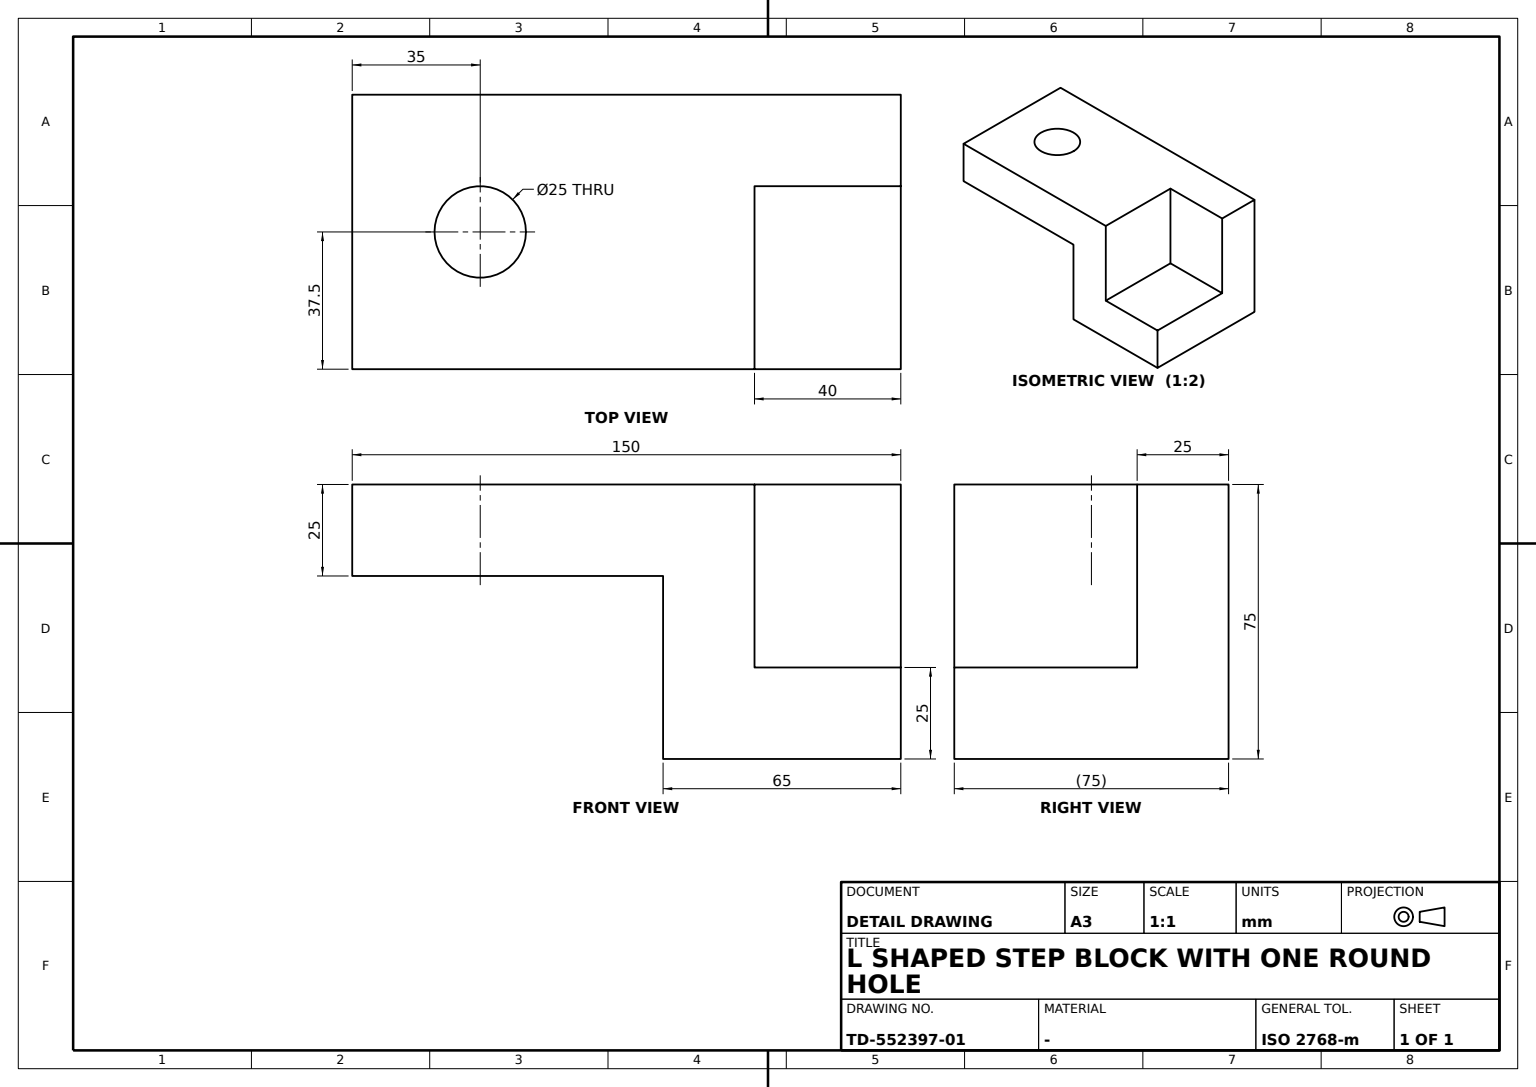
ISO-10303-21;
HEADER;
FILE_DESCRIPTION((''),'2;1');
FILE_NAME('','',(''),(''),'','','');
FILE_SCHEMA(('AUTOMOTIVE_DESIGN'));
ENDSEC;
DATA;
#10=SHAPE_REPRESENTATION_RELATIONSHIP('','',#262,#11);
#11=ADVANCED_BREP_SHAPE_REPRESENTATION('',(#260),#416);
#12=CIRCLE('',#268,12.5);
#13=CIRCLE('',#269,12.5);
#14=CIRCLE('',#274,12.5);
#15=CIRCLE('',#278,12.5);
#16=CYLINDRICAL_SURFACE('',#267,12.5);
#17=CYLINDRICAL_SURFACE('',#280,12.5);
#18=ORIENTED_EDGE('',*,*,#84,.F.);
#19=ORIENTED_EDGE('',*,*,#85,.F.);
#20=ORIENTED_EDGE('',*,*,#86,.T.);
#21=ORIENTED_EDGE('',*,*,#87,.T.);
#22=ORIENTED_EDGE('',*,*,#88,.T.);
#23=ORIENTED_EDGE('',*,*,#85,.T.);
#24=ORIENTED_EDGE('',*,*,#89,.T.);
#25=ORIENTED_EDGE('',*,*,#90,.F.);
#26=ORIENTED_EDGE('',*,*,#89,.F.);
#27=ORIENTED_EDGE('',*,*,#84,.T.);
#28=ORIENTED_EDGE('',*,*,#91,.F.);
#29=ORIENTED_EDGE('',*,*,#92,.F.);
#30=ORIENTED_EDGE('',*,*,#93,.F.);
#31=ORIENTED_EDGE('',*,*,#94,.F.);
#32=ORIENTED_EDGE('',*,*,#95,.F.);
#33=ORIENTED_EDGE('',*,*,#96,.F.);
#34=ORIENTED_EDGE('',*,*,#97,.F.);
#35=ORIENTED_EDGE('',*,*,#98,.F.);
#36=ORIENTED_EDGE('',*,*,#99,.F.);
#37=ORIENTED_EDGE('',*,*,#100,.F.);
#38=ORIENTED_EDGE('',*,*,#101,.F.);
#39=ORIENTED_EDGE('',*,*,#102,.F.);
#40=ORIENTED_EDGE('',*,*,#100,.T.);
#41=ORIENTED_EDGE('',*,*,#103,.F.);
#42=ORIENTED_EDGE('',*,*,#104,.F.);
#43=ORIENTED_EDGE('',*,*,#105,.T.);
#44=ORIENTED_EDGE('',*,*,#101,.T.);
#45=ORIENTED_EDGE('',*,*,#105,.F.);
#46=ORIENTED_EDGE('',*,*,#106,.F.);
#47=ORIENTED_EDGE('',*,*,#107,.T.);
#48=ORIENTED_EDGE('',*,*,#102,.T.);
#49=ORIENTED_EDGE('',*,*,#107,.F.);
#50=ORIENTED_EDGE('',*,*,#108,.F.);
#51=ORIENTED_EDGE('',*,*,#109,.T.);
#52=ORIENTED_EDGE('',*,*,#110,.T.);
#53=ORIENTED_EDGE('',*,*,#96,.T.);
#54=ORIENTED_EDGE('',*,*,#97,.T.);
#55=ORIENTED_EDGE('',*,*,#109,.F.);
#56=ORIENTED_EDGE('',*,*,#111,.F.);
#57=ORIENTED_EDGE('',*,*,#112,.T.);
#58=ORIENTED_EDGE('',*,*,#90,.T.);
#59=ORIENTED_EDGE('',*,*,#92,.T.);
#60=ORIENTED_EDGE('',*,*,#113,.T.);
#61=ORIENTED_EDGE('',*,*,#111,.T.);
#62=ORIENTED_EDGE('',*,*,#108,.T.);
#63=ORIENTED_EDGE('',*,*,#106,.T.);
#64=ORIENTED_EDGE('',*,*,#104,.T.);
#65=ORIENTED_EDGE('',*,*,#114,.T.);
#66=ORIENTED_EDGE('',*,*,#87,.F.);
#67=ORIENTED_EDGE('',*,*,#115,.T.);
#68=ORIENTED_EDGE('',*,*,#98,.T.);
#69=ORIENTED_EDGE('',*,*,#112,.F.);
#70=ORIENTED_EDGE('',*,*,#113,.F.);
#71=ORIENTED_EDGE('',*,*,#91,.T.);
#72=ORIENTED_EDGE('',*,*,#94,.T.);
#73=ORIENTED_EDGE('',*,*,#116,.T.);
#74=ORIENTED_EDGE('',*,*,#86,.F.);
#75=ORIENTED_EDGE('',*,*,#88,.F.);
#76=ORIENTED_EDGE('',*,*,#114,.F.);
#77=ORIENTED_EDGE('',*,*,#103,.T.);
#78=ORIENTED_EDGE('',*,*,#99,.T.);
#79=ORIENTED_EDGE('',*,*,#115,.F.);
#80=ORIENTED_EDGE('',*,*,#116,.F.);
#81=ORIENTED_EDGE('',*,*,#93,.T.);
#82=ORIENTED_EDGE('',*,*,#110,.F.);
#83=ORIENTED_EDGE('',*,*,#95,.T.);
#84=EDGE_CURVE('',#117,#118,#139,.T.);
#85=EDGE_CURVE('',#119,#117,#140,.T.);
#86=EDGE_CURVE('',#119,#120,#141,.T.);
#87=EDGE_CURVE('',#120,#118,#142,.T.);
#88=EDGE_CURVE('',#121,#119,#143,.T.);
#89=EDGE_CURVE('',#117,#122,#144,.T.);
#90=EDGE_CURVE('',#121,#122,#145,.T.);
#91=EDGE_CURVE('',#123,#118,#146,.T.);
#92=EDGE_CURVE('',#122,#123,#147,.T.);
#93=EDGE_CURVE('',#124,#125,#148,.T.);
#94=EDGE_CURVE('',#126,#124,#12,.T.);
#95=EDGE_CURVE('',#127,#126,#149,.F.);
#96=EDGE_CURVE('',#125,#127,#13,.T.);
#97=EDGE_CURVE('',#128,#129,#150,.T.);
#98=EDGE_CURVE('',#130,#128,#151,.T.);
#99=EDGE_CURVE('',#131,#130,#152,.T.);
#100=EDGE_CURVE('',#132,#131,#153,.T.);
#101=EDGE_CURVE('',#133,#132,#154,.T.);
#102=EDGE_CURVE('',#129,#133,#155,.T.);
#103=EDGE_CURVE('',#134,#131,#156,.T.);
#104=EDGE_CURVE('',#135,#134,#157,.T.);
#105=EDGE_CURVE('',#135,#132,#158,.T.);
#106=EDGE_CURVE('',#136,#135,#159,.T.);
#107=EDGE_CURVE('',#136,#133,#160,.T.);
#108=EDGE_CURVE('',#137,#136,#161,.T.);
#109=EDGE_CURVE('',#137,#129,#162,.T.);
#110=EDGE_CURVE('',#127,#125,#14,.T.);
#111=EDGE_CURVE('',#138,#137,#163,.T.);
#112=EDGE_CURVE('',#138,#128,#164,.T.);
#113=EDGE_CURVE('',#123,#138,#165,.T.);
#114=EDGE_CURVE('',#134,#121,#166,.T.);
#115=EDGE_CURVE('',#120,#130,#167,.T.);
#116=EDGE_CURVE('',#124,#126,#15,.T.);
#117=VERTEX_POINT('',#349);
#118=VERTEX_POINT('',#350);
#119=VERTEX_POINT('',#352);
#120=VERTEX_POINT('',#354);
#121=VERTEX_POINT('',#358);
#122=VERTEX_POINT('',#360);
#123=VERTEX_POINT('',#364);
#124=VERTEX_POINT('',#368);
#125=VERTEX_POINT('',#369);
#126=VERTEX_POINT('',#371);
#127=VERTEX_POINT('',#373);
#128=VERTEX_POINT('',#377);
#129=VERTEX_POINT('',#378);
#130=VERTEX_POINT('',#380);
#131=VERTEX_POINT('',#382);
#132=VERTEX_POINT('',#384);
#133=VERTEX_POINT('',#386);
#134=VERTEX_POINT('',#390);
#135=VERTEX_POINT('',#392);
#136=VERTEX_POINT('',#396);
#137=VERTEX_POINT('',#400);
#138=VERTEX_POINT('',#405);
#139=LINE('',#348,#168);
#140=LINE('',#351,#169);
#141=LINE('',#353,#170);
#142=LINE('',#355,#171);
#143=LINE('',#357,#172);
#144=LINE('',#359,#173);
#145=LINE('',#361,#174);
#146=LINE('',#363,#175);
#147=LINE('',#365,#176);
#148=LINE('',#367,#177);
#149=LINE('',#372,#178);
#150=LINE('',#376,#179);
#151=LINE('',#379,#180);
#152=LINE('',#381,#181);
#153=LINE('',#383,#182);
#154=LINE('',#385,#183);
#155=LINE('',#387,#184);
#156=LINE('',#389,#185);
#157=LINE('',#391,#186);
#158=LINE('',#393,#187);
#159=LINE('',#395,#188);
#160=LINE('',#397,#189);
#161=LINE('',#399,#190);
#162=LINE('',#401,#191);
#163=LINE('',#404,#192);
#164=LINE('',#406,#193);
#165=LINE('',#408,#194);
#166=LINE('',#409,#195);
#167=LINE('',#411,#196);
#168=VECTOR('',#285,1000.);
#169=VECTOR('',#286,1000.);
#170=VECTOR('',#287,1000.);
#171=VECTOR('',#288,1000.);
#172=VECTOR('',#291,1000.);
#173=VECTOR('',#292,1000.);
#174=VECTOR('',#293,1000.);
#175=VECTOR('',#296,1000.);
#176=VECTOR('',#297,1000.);
#177=VECTOR('',#300,1000.);
#178=VECTOR('',#303,1000.);
#179=VECTOR('',#308,1000.);
#180=VECTOR('',#309,1000.);
#181=VECTOR('',#310,1000.);
#182=VECTOR('',#311,1000.);
#183=VECTOR('',#312,1000.);
#184=VECTOR('',#313,1000.);
#185=VECTOR('',#316,1000.);
#186=VECTOR('',#317,1000.);
#187=VECTOR('',#318,1000.);
#188=VECTOR('',#321,1000.);
#189=VECTOR('',#322,1000.);
#190=VECTOR('',#325,1000.);
#191=VECTOR('',#326,1000.);
#192=VECTOR('',#331,1000.);
#193=VECTOR('',#332,1000.);
#194=VECTOR('',#335,1000.);
#195=VECTOR('',#336,1000.);
#196=VECTOR('',#339,1000.);
#197=EDGE_LOOP('',(#18,#19,#20,#21));
#198=EDGE_LOOP('',(#22,#23,#24,#25));
#199=EDGE_LOOP('',(#26,#27,#28,#29));
#200=EDGE_LOOP('',(#30,#31,#32,#33));
#201=EDGE_LOOP('',(#34,#35,#36,#37,#38,#39));
#202=EDGE_LOOP('',(#40,#41,#42,#43));
#203=EDGE_LOOP('',(#44,#45,#46,#47));
#204=EDGE_LOOP('',(#48,#49,#50,#51));
#205=EDGE_LOOP('',(#52,#53));
#206=EDGE_LOOP('',(#54,#55,#56,#57));
#207=EDGE_LOOP('',(#58,#59,#60,#61,#62,#63,#64,#65));
#208=EDGE_LOOP('',(#66,#67,#68,#69,#70,#71));
#209=EDGE_LOOP('',(#72,#73));
#210=EDGE_LOOP('',(#74,#75,#76,#77,#78,#79));
#211=EDGE_LOOP('',(#80,#81,#82,#83));
#212=FACE_BOUND('',#197,.T.);
#213=FACE_BOUND('',#198,.T.);
#214=FACE_BOUND('',#199,.T.);
#215=FACE_BOUND('',#200,.T.);
#216=FACE_BOUND('',#201,.T.);
#217=FACE_BOUND('',#202,.T.);
#218=FACE_BOUND('',#203,.T.);
#219=FACE_BOUND('',#204,.T.);
#220=FACE_BOUND('',#205,.T.);
#221=FACE_BOUND('',#206,.T.);
#222=FACE_BOUND('',#207,.T.);
#223=FACE_BOUND('',#208,.T.);
#224=FACE_BOUND('',#209,.T.);
#225=FACE_BOUND('',#210,.T.);
#226=FACE_BOUND('',#211,.T.);
#227=PLANE('',#264);
#228=PLANE('',#265);
#229=PLANE('',#266);
#230=PLANE('',#270);
#231=PLANE('',#271);
#232=PLANE('',#272);
#233=PLANE('',#273);
#234=PLANE('',#275);
#235=PLANE('',#276);
#236=PLANE('',#277);
#237=PLANE('',#279);
#238=ADVANCED_FACE('',(#212),#227,.T.);
#239=ADVANCED_FACE('',(#213),#228,.T.);
#240=ADVANCED_FACE('',(#214),#229,.T.);
#241=ADVANCED_FACE('',(#215),#16,.F.);
#242=ADVANCED_FACE('',(#216),#230,.F.);
#243=ADVANCED_FACE('',(#217),#231,.F.);
#244=ADVANCED_FACE('',(#218),#232,.F.);
#245=ADVANCED_FACE('',(#219,#220),#233,.F.);
#246=ADVANCED_FACE('',(#221),#234,.F.);
#247=ADVANCED_FACE('',(#222),#235,.T.);
#248=ADVANCED_FACE('',(#223,#224),#236,.F.);
#249=ADVANCED_FACE('',(#225),#237,.F.);
#250=ADVANCED_FACE('',(#226),#17,.F.);
#251=CLOSED_SHELL('',(#238,#239,#240,#241,#242,#243,#244,#245,#246,#247,#248,#249,#250));
#260=MANIFOLD_SOLID_BREP('',#251);
#261=SHAPE_DEFINITION_REPRESENTATION(#421,#262);
#262=SHAPE_REPRESENTATION('',(#263),#416);
#263=AXIS2_PLACEMENT_3D('',#346,#281,#282);
#264=AXIS2_PLACEMENT_3D('',#347,#283,#284);
#265=AXIS2_PLACEMENT_3D('',#356,#289,#290);
#266=AXIS2_PLACEMENT_3D('',#362,#294,#295);
#267=AXIS2_PLACEMENT_3D('',#366,#298,#299);
#268=AXIS2_PLACEMENT_3D('',#370,#301,#302);
#269=AXIS2_PLACEMENT_3D('',#374,#304,#305);
#270=AXIS2_PLACEMENT_3D('',#375,#306,#307);
#271=AXIS2_PLACEMENT_3D('',#388,#314,#315);
#272=AXIS2_PLACEMENT_3D('',#394,#319,#320);
#273=AXIS2_PLACEMENT_3D('',#398,#323,#324);
#274=AXIS2_PLACEMENT_3D('',#402,#327,#328);
#275=AXIS2_PLACEMENT_3D('',#403,#329,#330);
#276=AXIS2_PLACEMENT_3D('',#407,#333,#334);
#277=AXIS2_PLACEMENT_3D('',#410,#337,#338);
#278=AXIS2_PLACEMENT_3D('',#412,#340,#341);
#279=AXIS2_PLACEMENT_3D('',#413,#342,#343);
#280=AXIS2_PLACEMENT_3D('',#414,#344,#345);
#281=DIRECTION('',(0.,0.,1.));
#282=DIRECTION('',(1.,0.,0.));
#283=DIRECTION('',(0.,-1.,0.));
#284=DIRECTION('',(0.,0.,-1.));
#285=DIRECTION('',(0.,0.,1.));
#286=DIRECTION('',(-1.,0.,0.));
#287=DIRECTION('',(0.,0.,1.));
#288=DIRECTION('',(-1.,0.,0.));
#289=DIRECTION('',(0.,0.,1.));
#290=DIRECTION('',(1.,0.,0.));
#291=DIRECTION('',(0.,1.,0.));
#292=DIRECTION('',(0.,-1.,0.));
#293=DIRECTION('',(-1.,0.,0.));
#294=DIRECTION('',(1.,0.,0.));
#295=DIRECTION('',(0.,0.,-1.));
#296=DIRECTION('',(0.,1.,0.));
#297=DIRECTION('',(0.,0.,1.));
#298=DIRECTION('',(-9.25185853854297E-17,0.,-1.));
#299=DIRECTION('',(-1.,0.,0.));
#300=DIRECTION('',(-9.25185853854297E-17,0.,-1.));
#301=DIRECTION('',(-9.25185853854297E-17,0.,-1.));
#302=DIRECTION('',(-1.,0.,0.));
#303=DIRECTION('',(-9.25185853854297E-17,0.,-1.));
#304=DIRECTION('',(0.,0.,1.));
#305=DIRECTION('',(1.,0.,0.));
#306=DIRECTION('',(0.,-1.,0.));
#307=DIRECTION('',(0.,0.,-1.));
#308=DIRECTION('',(-1.11022302462516E-15,0.,-1.));
#309=DIRECTION('',(-1.,0.,9.25185853854297E-17));
#310=DIRECTION('',(-2.77555756156289E-17,0.,1.));
#311=DIRECTION('',(1.,0.,8.32667268468867E-17));
#312=DIRECTION('',(0.,0.,-1.));
#313=DIRECTION('',(1.,0.,0.));
#314=DIRECTION('',(-8.32667268468867E-17,0.,1.));
#315=DIRECTION('',(1.,0.,8.32667268468867E-17));
#316=DIRECTION('',(0.,1.,0.));
#317=DIRECTION('',(1.,0.,8.32667268468867E-17));
#318=DIRECTION('',(0.,1.,0.));
#319=DIRECTION('',(1.,0.,0.));
#320=DIRECTION('',(0.,0.,-1.));
#321=DIRECTION('',(0.,0.,-1.));
#322=DIRECTION('',(0.,1.,0.));
#323=DIRECTION('',(0.,0.,1.));
#324=DIRECTION('',(1.,0.,0.));
#325=DIRECTION('',(1.,0.,0.));
#326=DIRECTION('',(0.,1.,0.));
#327=DIRECTION('',(0.,0.,1.));
#328=DIRECTION('',(1.,0.,0.));
#329=DIRECTION('',(1.,0.,-1.11022302462516E-15));
#330=DIRECTION('',(-1.11022302462516E-15,0.,-1.));
#331=DIRECTION('',(-1.11022302462516E-15,0.,-1.));
#332=DIRECTION('',(0.,1.,0.));
#333=DIRECTION('',(0.,-1.,0.));
#334=DIRECTION('',(0.,0.,-1.));
#335=DIRECTION('',(-1.,0.,9.25185853854297E-17));
#336=DIRECTION('',(-2.77555756156289E-17,0.,1.));
#337=DIRECTION('',(-9.25185853854297E-17,0.,-1.));
#338=DIRECTION('',(-1.,0.,9.25185853854297E-17));
#339=DIRECTION('',(0.,1.,0.));
#340=DIRECTION('',(-9.25185853854297E-17,0.,-1.));
#341=DIRECTION('',(-1.,0.,0.));
#342=DIRECTION('',(-1.,0.,-2.77555756156289E-17));
#343=DIRECTION('',(-2.77555756156289E-17,0.,1.));
#344=DIRECTION('',(-9.25185853854297E-17,0.,-1.));
#345=DIRECTION('',(-1.,0.,0.));
#346=CARTESIAN_POINT('',(0.,0.,0.));
#347=CARTESIAN_POINT('',(0.,-25.,0.));
#348=CARTESIAN_POINT('',(-40.,-25.,75.));
#349=CARTESIAN_POINT('',(-40.,-25.,25.));
#350=CARTESIAN_POINT('',(-40.,-25.,75.));
#351=CARTESIAN_POINT('',(-40.,-25.,25.));
#352=CARTESIAN_POINT('',(0.,-25.,25.));
#353=CARTESIAN_POINT('',(-2.08166817117217E-15,-25.,25.));
#354=CARTESIAN_POINT('',(-2.08166817117217E-15,-25.,75.));
#355=CARTESIAN_POINT('',(0.,-25.,75.));
#356=CARTESIAN_POINT('',(-40.,-150.,25.));
#357=CARTESIAN_POINT('',(0.,-150.,25.));
#358=CARTESIAN_POINT('',(0.,-75.,25.));
#359=CARTESIAN_POINT('',(-40.,-150.,25.));
#360=CARTESIAN_POINT('',(-40.,-75.,25.));
#361=CARTESIAN_POINT('',(0.,-75.,25.));
#362=CARTESIAN_POINT('',(-40.,-150.,75.));
#363=CARTESIAN_POINT('',(-40.,-150.,75.));
#364=CARTESIAN_POINT('',(-40.,-75.,75.));
#365=CARTESIAN_POINT('',(-40.,-75.,0.));
#366=CARTESIAN_POINT('',(-115.,-37.5,75.));
#367=CARTESIAN_POINT('',(-102.5,-37.5,75.));
#368=CARTESIAN_POINT('',(-102.5,-37.5,75.));
#369=CARTESIAN_POINT('',(-102.5,-37.5,50.));
#370=CARTESIAN_POINT('',(-115.,-37.5,75.));
#371=CARTESIAN_POINT('',(-127.5,-37.5,75.));
#372=CARTESIAN_POINT('',(-127.5,-37.5,75.));
#373=CARTESIAN_POINT('',(-127.5,-37.5,50.));
#374=CARTESIAN_POINT('',(-115.,-37.5,50.));
#375=CARTESIAN_POINT('',(0.,0.,0.));
#376=CARTESIAN_POINT('',(-150.,0.,75.));
#377=CARTESIAN_POINT('',(-150.,0.,75.));
#378=CARTESIAN_POINT('',(-150.,0.,50.));
#379=CARTESIAN_POINT('',(0.,0.,75.));
#380=CARTESIAN_POINT('',(-2.08166817117217E-15,0.,75.));
#381=CARTESIAN_POINT('',(0.,0.,0.));
#382=CARTESIAN_POINT('',(0.,0.,-1.73472347597681E-15));
#383=CARTESIAN_POINT('',(-65.,0.,-7.14706072102445E-15));
#384=CARTESIAN_POINT('',(-65.,0.,0.));
#385=CARTESIAN_POINT('',(-65.,0.,50.));
#386=CARTESIAN_POINT('',(-65.,0.,50.));
#387=CARTESIAN_POINT('',(-150.,0.,50.));
#388=CARTESIAN_POINT('',(-65.,-75.,-7.14706072102445E-15));
#389=CARTESIAN_POINT('',(0.,-75.,-1.73472347597681E-15));
#390=CARTESIAN_POINT('',(0.,-75.,-1.73472347597681E-15));
#391=CARTESIAN_POINT('',(-65.,-75.,-7.14706072102445E-15));
#392=CARTESIAN_POINT('',(-65.,-75.,0.));
#393=CARTESIAN_POINT('',(-65.,-75.,0.));
#394=CARTESIAN_POINT('',(-65.,-75.,50.));
#395=CARTESIAN_POINT('',(-65.,-75.,50.));
#396=CARTESIAN_POINT('',(-65.,-75.,50.));
#397=CARTESIAN_POINT('',(-65.,-75.,50.));
#398=CARTESIAN_POINT('',(-150.,-75.,50.));
#399=CARTESIAN_POINT('',(-150.,-75.,50.));
#400=CARTESIAN_POINT('',(-150.,-75.,50.));
#401=CARTESIAN_POINT('',(-150.,-75.,50.));
#402=CARTESIAN_POINT('',(-115.,-37.5,50.));
#403=CARTESIAN_POINT('',(-150.,-75.,75.));
#404=CARTESIAN_POINT('',(-150.,-75.,75.));
#405=CARTESIAN_POINT('',(-150.,-75.,75.));
#406=CARTESIAN_POINT('',(-150.,-75.,75.));
#407=CARTESIAN_POINT('',(0.,-75.,0.));
#408=CARTESIAN_POINT('',(0.,-75.,75.));
#409=CARTESIAN_POINT('',(0.,-75.,0.));
#410=CARTESIAN_POINT('',(0.,-75.,75.));
#411=CARTESIAN_POINT('',(-2.08166817117217E-15,-75.,75.));
#412=CARTESIAN_POINT('',(-115.,-37.5,75.));
#413=CARTESIAN_POINT('',(0.,-75.,0.));
#414=CARTESIAN_POINT('',(-115.,-37.5,75.));
#416=(GEOMETRIC_REPRESENTATION_CONTEXT(3)GLOBAL_UNCERTAINTY_ASSIGNED_CONTEXT((#417))GLOBAL_UNIT_ASSIGNED_CONTEXT((#420,#419,#418))REPRESENTATION_CONTEXT('export','TOP_LEVEL_ASSEMBLY_PART'));
#417=UNCERTAINTY_MEASURE_WITH_UNIT(LENGTH_MEASURE(0.005),#420,'DISTANCE_ACCURACY_VALUE','Maximum Tolerance applied to model');
#418=(NAMED_UNIT(*)SI_UNIT($,.STERADIAN.)SOLID_ANGLE_UNIT());
#419=(NAMED_UNIT(*)PLANE_ANGLE_UNIT()SI_UNIT($,.RADIAN.));
#420=(LENGTH_UNIT()NAMED_UNIT(*)SI_UNIT(.MILLI.,.METRE.));
#421=PRODUCT_DEFINITION_SHAPE('','',#422);
#422=PRODUCT_DEFINITION('','',#424,#423);
#423=PRODUCT_DEFINITION_CONTEXT('',#430,'design');
#424=PRODUCT_DEFINITION_FORMATION_WITH_SPECIFIED_SOURCE('','',#426,.NOT_KNOWN.);
#425=PRODUCT_RELATED_PRODUCT_CATEGORY('','',(#426));
#426=PRODUCT('','','',(#428));
#427=PRODUCT_CATEGORY('','');
#428=PRODUCT_CONTEXT('',#430,'mechanical');
#429=APPLICATION_PROTOCOL_DEFINITION('international standard','ap242_managed_model_based_3d_engineering',2011,#430);
#430=APPLICATION_CONTEXT('managed model based 3d engineering');
ENDSEC;
END-ISO-10303-21;
